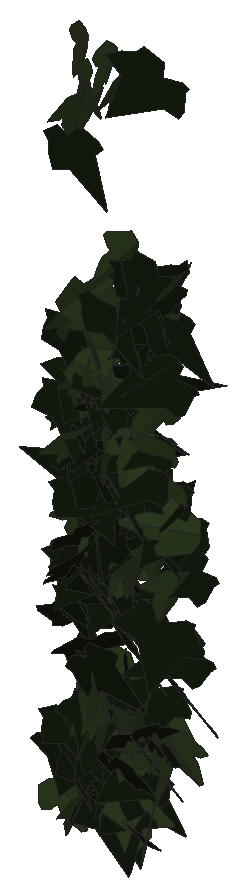
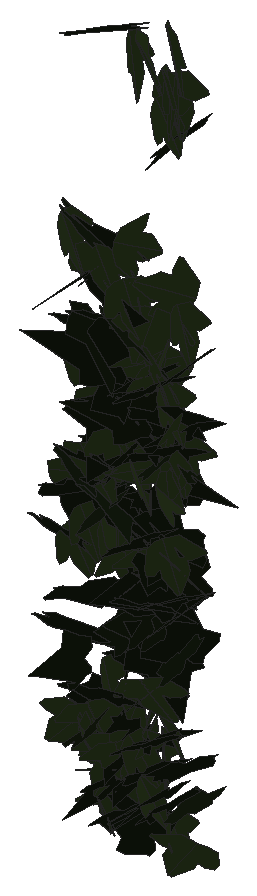
# SketchUp Ruby script. Lengths in inches.
U = 1.inch
M = Sketchup.active_model
def pt(a) = Geom::Point3d.new(a.map { |v| v * U })
def face(e, loops, mat)
  f = e.add_face(loops[0].map { |a| pt(a) })
  loops[1..].each { |l| e.add_face(l.map { |a| pt(a) }).erase! }
  f.material = f.back_material = mat if mat
  f
end
# faces: each face lists its corners as indices into pts; further lists are holes
def faces(e, pts, list, mat = nil) = list.each { |f| face(e, (f[0].is_a?(Array) ? f : [f]).map { |l| l.map { |i| pts[i] } }, mat) }
# xy, xz, yz: faces in a plane at the given z, y or x. An outline is a flat list of corners, or four numbers for a rectangle; further outlines are holes
def ring(l) = l.size == 4 ? [[l[0], l[1]], [l[2], l[1]], [l[2], l[3]], [l[0], l[3]]] : l.each_slice(2).to_a
def flat(e, list, mat, &to3) = list.each { |f| face(e, (f[0].is_a?(Array) ? f : [f]).map { |l| ring(l).map { |u, v| to3.(u, v) } }, mat) }
def xy(e, z, list, mat = nil) = flat(e, list, mat) { |x, y| [x, y, z] }
def xz(e, y, list, mat = nil) = flat(e, list, mat) { |x, z| [x, y, z] }
def yz(e, x, list, mat = nil) = flat(e, list, mat) { |y, z| [x, y, z] }
def lines(e, pts, list) = list.each { |a, b| e.add_line(pt(pts[a]), pt(pts[b])) }
# prism: a flat outline (further loops are holes) pulled along v
def prism(e, loops, v, mat = nil)
  f = face(e, loops, mat); d = Geom::Vector3d.new(v.map { |x| x * U })
  f.pushpull(f.normal.samedirection?(d) ? d.length : -d.length)
end
def box(e, o, s, mat = nil) = prism(e, [[o, [o[0] + s[0], o[1], o[2]], [o[0] + s[0], o[1] + s[1], o[2]], [o[0], o[1] + s[1], o[2]]]], [0, 0, s[2]], mat)
def at(x, y, z, deg = 0) = Geom::Transformation.translation(pt([x, y, z])) * Geom::Transformation.rotation(ORIGIN, Z_AXIS, deg.degrees)
def axes(o, x, y, z) = Geom::Transformation.new([*x, 0, *y, 0, *z, 0, *pt(o).to_a, 1])
def part(name) = M.definitions.add(name)
# library, detail: a bought-in or finely detailed component or shape, given as its bounding box
def library(name, o, s) = part(name).tap { |d| box(d.entities, o, s) }
def detail(e, o, s) = box(e.add_group.entities, o, s)
def put(e, d, t, mat = nil) = e.add_instance(d, t).tap { |i| i.material = mat if mat }
def group(e, t, mat = nil) = e.add_group.tap { |g| g.transformation = t; g.material = mat if mat }.entities
root = M.entities
M.materials.add("1026 AP 7946 SUNNY SIDE UP").color = [254, 231, 186]
M.materials.add("efeu1").color = [18, 25, 13]
M.materials.add("efeu2").color = [43, 57, 29]
c1 = part("ivyleaf_9")
p = [[1.54,2.16,1.25],[1.36,2.04,1.19],[-0.21,0.99,0.68],[-0.71,1.11,0.82],[-0.85,0.86,0.67],[-0.8,0.17,0.21],
  [-0.9,-0.01,0.1],[-0.67,-0.16,-0.02],[-0.08,-0.08,-0.05],[-0.03,-0.6,-0.4],[0.65,-0.88,-0.66],[0.83,-0.6,-0.49],
  [1.29,-0.42,-0.43],[1.8125,-0.07,-0.26],[1.21,0.44,0.15]]
faces(c1.entities,p,[[0,1,2,3,4,5,6,7,8,9,10,11,12,13,14]],"efeu1")
c2 = part("ivyleaf_10")
p = [[0,0.5,-0.03],[-0.0625,2.02,-0.43],[-0.19,2.01,-0.46],[-0.54,1.05,-0.29],[-0.52,0.625,-0.18],[-0.83,0.76,-0.28],
  [-1.16,0.64,-0.33],[-1.15,0.33,-0.24],[-0.77,-0.39,0.02],[-0.3,-0.51,0.16],[0.04,-0.48,0.23],[-0.02,2.01,-0.4375],
  [-0.06,2.01,-0.43],[0.04,-0.49,0.23],[0.67,-0.49,0.14],[1.38,0.36,-0.2],[1.375,0.51,-0.24],[0.81,0.65,-0.19],
  [0.62,0.59,-0.15],[0.6,1.09,-0.28],[0.5,1.23,-0.31]]
faces(c2.entities,p,[[0,1,2,3,4,5,6,7,8,9,10],[11,12,0,13,14,15,16,17,18,19,20]],"efeu2")
put(root,c1,axes([118.58,212.68,268.59],[-0.10148,-0.2145,0.16727],[0.05063,-0.17313,-0.22179],[0.42114,-0.03087,0.06697]),"1026 AP 7946 SUNNY SIDE UP")
put(root,c2,axes([118.54,212.65,268.07],[0.32447,0.10776,0.11567],[0.15112,0.05714,-0.23942],[-0.19158,0.22757,0.00705]),"1026 AP 7946 SUNNY SIDE UP")
put(root,c2,axes([118.68,212.77,274.12],[-0.06073,0.27731,-0.0585],[0.00468,-0.0585,-0.28874],[-0.44557,-0.03841,0.00494]),"1026 AP 7946 SUNNY SIDE UP")
put(root,c1,axes([118.59,212.76,274.85],[0.03448,-0.29512,0.03283],[-0.01092,-0.03414,-0.30491],[0.46691,0.021,-0.00956]),"1026 AP 7946 SUNNY SIDE UP")
put(root,c2,axes([118.8,212.83,272.25],[-0.18056,-0.25267,0.05829],[0.00801,-0.06563,-0.2845],[0.40755,-0.11065,0.03141]),"1026 AP 7946 SUNNY SIDE UP")
put(root,c2,axes([118.81,212.51,275.38],[-0.01092,-0.29639,-0.03515],[-0.00326,0.03249,-0.30522],[0.46882,-0.00667,-0.00294]),"1026 AP 7946 SUNNY SIDE UP")
put(root,c1,axes([118.55,212.8125,270.79],[0.18485,-0.24588,0.0457],[0.01515,-0.04607,-0.2808],[0.39297,0.11743,-0.01067]),"1026 AP 7946 SUNNY SIDE UP")
put(root,c1,axes([118.61,212.83,271.41],[0.05177,-0.27805,0.00823],[0.0003,-0.00961,-0.2885],[0.43746,0.03291,-0.00078]),"1026 AP 7946 SUNNY SIDE UP")
put(root,c2,axes([118.83,212.76,274.35],[0.00803,-0.29251,0.01042],[-0.01331,-0.01192,-0.30133],[0.46013,0.00476,-0.0089]),"1026 AP 7946 SUNNY SIDE UP")
put(root,c2,axes([118.9,212.65,278.67],[-0.31786,0.21972,0.09851],[-0.14415,0.04293,-0.30501],[-0.34729,-0.21892,0.03644]),"1026 AP 7946 SUNNY SIDE UP")
put(root,c1,axes([118.69,212.68,273.9],[-0.09442,-0.28697,-0.00864],[0.02044,0.00418,-0.30176],[0.45089,-0.06028,0.01187]),"1026 AP 7946 SUNNY SIDE UP")
put(root,c1,axes([118.91,212.89,274.19],[-0.3765,-0.16155,0.02026],[-0.00418,-0.03272,-0.29659],[0.25605,-0.23809,0.02495]),"1026 AP 7946 SUNNY SIDE UP")
put(root,c1,axes([118.6875,212.63,269.2],[0.01907,-0.25324,-0.11669],[0.04147,0.11249,-0.25882],[0.43332,0.00038,0.0299]),"1026 AP 7946 SUNNY SIDE UP")
put(root,c2,axes([118.9,212.44,273.5],[-0.12951,-0.28312,-0.0189],[0.01697,0.01429,-0.3036],[0.44563,-0.08283,0.00607]),"1026 AP 7946 SUNNY SIDE UP")
put(root,c2,axes([118.91,212.66,278.73],[0.19427,-0.27639,-0.07992],[-0.02868,0.07502,-0.31114],[0.44982,0.12415,0.01468]),"1026 AP 7946 SUNNY SIDE UP")
put(root,c2,axes([118.9,212.77,278.38],[0.00487,-0.30093,0.07367],[0.02675,-0.07295,-0.31003],[0.48625,0.00703,0.01632]),"1026 AP 7946 SUNNY SIDE UP")
put(root,c2,axes([118.91,212.58,279.31],[0.25386,-0.26163,-0.09519],[-0.02226,0.0973,-0.31379],[0.43496,0.15768,0.0395]),"1026 AP 7946 SUNNY SIDE UP")
put(root,c1,axes([118.9,212.77,271.46],[-0.25139,-0.19979,0.10642],[-0.01696,-0.1211,-0.25639],[0.35407,-0.14765,0.06328]),"1026 AP 7946 SUNNY SIDE UP")
put(root,c1,axes([118.85,212.57,270.75],[0.36294,0.1012,0.16315],[-0.24909,-0.02853,0.2574],[0.1576,-0.27814,0.0311]),"1026 AP 7946 SUNNY SIDE UP")
put(root,c2,axes([118.95,212.43,278.55],[-0.04065,-0.30751,-0.04097],[0.01889,0.03713,-0.31756],[0.48684,-0.02712,0.0089]),"1026 AP 7946 SUNNY SIDE UP")
put(root,c1,axes([119.32,212.4,273.06],[-0.2342,-0.03979,-0.26199],[-0.37431,-0.08981,0.15772],[-0.15306,0.2805,0.01517]),"1026 AP 7946 SUNNY SIDE UP")
put(root,c2,axes([118.89,212.77,273.02],[0.11866,-0.1923,0.20503],[0.10479,-0.18876,-0.21385],[0.42362,0.10055,-0.00453]),"1026 AP 7946 SUNNY SIDE UP")
put(root,c2,axes([118.98,212.4375,268.15],[0.03323,-0.2702,0.01416],[0.00097,-0.01527,-0.2793],[0.42554,0.02114,-0.00047]),"1026 AP 7946 SUNNY SIDE UP")
put(root,c1,axes([118.99,212.83,273.55],[-0.26978,-0.23022,0.03448],[-0.00865,-0.03917,-0.29538],[0.366,-0.17062,0.01843]),"1026 AP 7946 SUNNY SIDE UP")
put(root,c1,axes([118.84,212.17,271.6],[0.19476,0.04727,0.25703],[0.24352,0.20557,-0.11826],[-0.3159,0.18761,0.0673]),"1026 AP 7946 SUNNY SIDE UP")
put(root,c1,axes([118.87,212.7,268.61],[0.02193,-0.27626,-0.0293],[-0.01072,0.02655,-0.28476],[0.43632,0.01454,-0.00552]),"1026 AP 7946 SUNNY SIDE UP")
put(root,c1,axes([118.85,212.42,277.9375],[0.13716,-0.27594,-0.10569],[-0.04552,0.0968,-0.29757],[0.45981,0.0919,0.00207]),"1026 AP 7946 SUNNY SIDE UP")
put(root,c1,axes([119.17,212.46,270.58],[0.06548,0.26201,-0.10257],[-0.03676,-0.09857,-0.27379],[-0.44004,0.04722,0.00761]),"1026 AP 7946 SUNNY SIDE UP")
put(root,c1,axes([119.01,212.26,273.3],[-0.19086,0.27196,-0.01341],[0.00514,0.01739,0.30674],[0.42821,0.12101,-0.00966]),"1026 AP 7946 SUNNY SIDE UP")
put(root,c1,axes([119.04,212.26,272.2],[0.18811,0.23917,0.09452],[0.07675,0.0766,-0.2749],[-0.39464,0.1289,-0.00841]),"1026 AP 7946 SUNNY SIDE UP")
put(root,c2,axes([118.99,212.32,275.57],[-0.03665,-0.15773,0.27901],[0.03852,0.27073,0.16564],[-0.49253,0.03291,-0.00781]),"1026 AP 7946 SUNNY SIDE UP")
put(root,c1,axes([119.17,212.65,271.99],[-0.1635,0.17125,-0.20163],[0.12844,-0.17971,-0.20672],[-0.38944,-0.13116,0.01647]),"1026 AP 7946 SUNNY SIDE UP")
put(root,c1,axes([119.28,212.65,272.125],[-0.41933,0.08612,-0.02938],[0.02968,-0.03548,-0.28749],[-0.13977,-0.2659,0.0271]),"1026 AP 7946 SUNNY SIDE UP")
put(root,c2,axes([119.05,212.68,273.6],[0.42207,-0.09618,-0.00233],[-0.01596,-0.02327,-0.29272],[0.15041,0.26742,-0.02452]),"1026 AP 7946 SUNNY SIDE UP")
put(root,c2,axes([119.125,212.8125,270.22],[0.36804,0.09952,-0.10881],[-0.14682,-0.05156,-0.26212],[-0.17553,0.2518,-0.0089]),"1026 AP 7946 SUNNY SIDE UP")
put(root,c2,axes([119.12,212.81,268.79],[0.02146,-0.25286,0.07339],[0.00072,-0.07275,-0.26128],[0.41369,0.01324,-0.00335]),"1026 AP 7946 SUNNY SIDE UP")
put(root,c1,axes([118.92,212.7,268.75],[0.18081,-0.19196,-0.17184],[-0.04871,0.16996,-0.22397],[0.39576,0.10862,0.05094]),"1026 AP 7946 SUNNY SIDE UP")
put(root,c1,axes([119.13,212.82,269.02],[-0.19573,-0.20834,0.09507],[-0.06147,-0.08544,-0.25033],[0.35375,-0.13012,0.0091]),"1026 AP 7946 SUNNY SIDE UP")
put(root,c1,axes([118.97,212.89,270.26],[0.03992,-0.26487,0.05518],[-0.00324,-0.0555,-0.27434],[0.42538,0.02443,-0.00727]),"1026 AP 7946 SUNNY SIDE UP")
put(root,c1,axes([118.87,212.83,271.2],[0.24445,-0.2175,0.07178],[0.04949,-0.06458,-0.27554],[0.35629,0.1582,-0.01097]),"1026 AP 7946 SUNNY SIDE UP")
put(root,c2,axes([119.16,212.41,269.27],[0.10542,-0.24459,-0.1297],[-0.00143,0.12797,-0.25874],[0.43156,0.06017,0.03083]),"1026 AP 7946 SUNNY SIDE UP")
put(root,c1,axes([118.93,212.6875,273.5],[0.26532,-0.2202,-0.0903],[-0.04809,0.08493,-0.28402],[0.36882,0.16948,0.02792]),"1026 AP 7946 SUNNY SIDE UP")
put(root,c2,axes([119.27,212.66,274.74],[0.20544,-0.20687,-0.15928],[-0.15272,0.11978,-0.25086],[0.3751,0.16207,-0.0149]),"1026 AP 7946 SUNNY SIDE UP")
put(root,c2,axes([119.09,212.54,274.94],[-0.21051,0.25398,-0.05746],[0.03298,-0.05361,-0.29601],[-0.40804,-0.13536,0.00572]),"1026 AP 7946 SUNNY SIDE UP")
put(root,c2,axes([119.23,212.39,269.61],[0.25938,-0.20632,-0.07883],[-0.09868,0.04603,-0.27112],[0.33098,0.17541,-0.01905]),"1026 AP 7946 SUNNY SIDE UP")
put(root,c1,axes([119.13,212.65,269.4],[-0.16533,-0.24244,0.04077],[-0.00673,-0.04272,-0.27216],[0.38655,-0.10444,0.0127]),"1026 AP 7946 SUNNY SIDE UP")
put(root,c1,axes([119.18,212.85,271.35],[-0.33244,-0.1684,-0.06579],[0.12306,0.00121,-0.27428],[0.25447,-0.22058,0.04668]),"1026 AP 7946 SUNNY SIDE UP")
put(root,c1,axes([119.09,212.91,269.47],[-0.10931,-0.25655,0.01204],[0.04968,-0.02205,-0.2714],[0.40086,-0.06722,0.03692]),"1026 AP 7946 SUNNY SIDE UP")
put(root,c1,axes([119.14,212.8125,274.4],[-0.15244,-0.27137,0.05732],[0.00506,-0.06167,-0.29625],[0.43604,-0.09416,0.02347]),"1026 AP 7946 SUNNY SIDE UP")
put(root,c2,axes([119.18,212.66,275.29],[-0.3818,-0.16452,-0.06141],[0.12487,-0.01448,-0.29679],[0.24463,-0.24938,0.05565]),"1026 AP 7946 SUNNY SIDE UP")
put(root,c2,axes([119.1875,212.6,274.59],[0.06134,0.27653,-0.08104],[-0.05979,-0.07531,-0.28689],[-0.44879,0.04783,0.02714]),"1026 AP 7946 SUNNY SIDE UP")
put(root,c2,axes([118.94,212.64,273.3],[-0.13355,-0.07805,-0.27428],[0.39461,0.09604,-0.11111],[0.18444,-0.26199,0.0391]),"1026 AP 7946 SUNNY SIDE UP")
put(root,c2,axes([119.21,212.76,279.11],[0.27061,-0.25999,0.04793],[0.02709,-0.04613,-0.32128],[0.41484,0.17261,-0.01028]),"1026 AP 7946 SUNNY SIDE UP")
put(root,c2,axes([119.3,212.8,269.32],[-0.05993,-0.25485,0.08837],[-0.02874,-0.08545,-0.26591],[0.42257,-0.04196,-0.00555]),"1026 AP 7946 SUNNY SIDE UP")
put(root,c2,axes([119.26,212.51,274.42],[0.33919,-0.18615,-0.03514],[-0.0489,0.01453,-0.2933],[0.29324,0.21775,-0.00826]),"1026 AP 7946 SUNNY SIDE UP")
put(root,c2,axes([119.1875,212.68,272.01],[0.20738,0.2401,-0.04856],[-0.01317,-0.05063,-0.28198],[-0.38493,0.13109,-0.01651]),"1026 AP 7946 SUNNY SIDE UP")
put(root,c1,axes([118.96,212.65,271.63],[0.4236,-0.02141,0.0859],[0.12889,-0.02116,-0.27816],[0.04195,0.28124,-0.01272]),"1026 AP 7946 SUNNY SIDE UP")
put(root,c1,axes([119.06,212.46,272.82],[-0.0129,-0.23668,-0.17327],[0.10554,0.16081,-0.23747],[0.44292,-0.04521,0.05154]),"1026 AP 7946 SUNNY SIDE UP")
put(root,c2,axes([119.33,212.4,269.41],[0.07074,-0.07671,-0.27977],[0.02194,0.27483,-0.07611],[0.44252,-0.00136,0.04849]),"1026 AP 7946 SUNNY SIDE UP")
put(root,c2,axes([119.33,212.76,273.21],[0.14434,-0.2762,0.01395],[0.00846,-0.01413,-0.29992],[0.43487,0.09195,0.0012]),"1026 AP 7946 SUNNY SIDE UP")
put(root,c1,axes([119.59,212.28,272.02],[-0.04798,0.10117,0.30367],[-0.20254,0.26497,-0.10608],[-0.44528,-0.13142,0.01553]),"1026 AP 7946 SUNNY SIDE UP")
put(root,c2,axes([119.51,212.39,273.15],[-0.24806,0.15581,0.2064],[-0.2529,0.11977,-0.22673],[-0.30731,-0.22434,0.01998]),"1026 AP 7946 SUNNY SIDE UP")
put(root,c2,axes([119.3,212.34,269.9375],[0.11206,-0.21982,-0.16627],[0.08462,0.17368,-0.2199],[0.41919,0.0237,0.08884]),"1026 AP 7946 SUNNY SIDE UP")
put(root,c1,axes([119.48,212.57,274.16],[0.13879,0.25151,-0.1236],[-0.1024,-0.10528,-0.27408],[-0.42704,0.10699,0.02555]),"1026 AP 7946 SUNNY SIDE UP")
put(root,c1,axes([119.26,212.67,274.46],[-0.03376,-0.29447,-0.02081],[0.01633,0.01781,-0.30392],[0.46366,-0.02207,0.00919]),"1026 AP 7946 SUNNY SIDE UP")
put(root,c2,axes([119.13,212.42,274.64],[-0.14289,-0.11409,-0.26965],[0.39928,0.09191,-0.13188],[0.20326,-0.26074,0.06949]),"1026 AP 7946 SUNNY SIDE UP")
put(root,c1,axes([119.15,212.75,271.13],[0.26787,-0.2088,0.06411],[0.03774,-0.06203,-0.27721],[0.34105,0.17087,-0.01968]),"1026 AP 7946 SUNNY SIDE UP")
put(root,c2,axes([119.47,212.76,275.63],[-0.20217,-0.26545,0.06075],[0.0069,-0.0689,-0.30232],[0.42803,-0.12427,0.03357]),"1026 AP 7946 SUNNY SIDE UP")
put(root,c1,axes([119.375,212.83,272.15],[-0.17087,-0.24373,0.09093],[-0.02084,-0.09185,-0.27434],[0.40781,-0.10682,0.02408]),"1026 AP 7946 SUNNY SIDE UP")
put(root,c2,axes([119.45,212.82,276.32],[-0.00921,-0.12799,0.29569],[0.05921,-0.28602,-0.13195],[0.49165,0.03205,0.02143]),"1026 AP 7946 SUNNY SIDE UP")
put(root,c1,axes([119.32,212.74,273.52],[0.13451,-0.24198,-0.13025],[-0.08259,0.11397,-0.26352],[0.42026,0.09984,-0.0101]),"1026 AP 7946 SUNNY SIDE UP")
put(root,c1,axes([119.3,212.75,271.62],[0.06004,-0.27427,0.04607],[0.0032,-0.04643,-0.28552],[0.43735,0.038,-0.00423]),"1026 AP 7946 SUNNY SIDE UP")
put(root,c1,axes([119.72,212.73,275.18],[-0.34567,0.19063,-0.03887],[0.01916,-0.04497,-0.29885],[-0.3053,-0.21866,0.02526]),"1026 AP 7946 SUNNY SIDE UP")
put(root,c2,axes([119.53,212.57,278.99],[0.07579,-0.30265,-0.08662],[0.01276,0.08451,-0.31451],[0.49303,0.04434,0.02145]),"1026 AP 7946 SUNNY SIDE UP")
put(root,c1,axes([119.16,212.42,270.3],[0.0599,-0.06791,-0.27882],[0.41852,0.08966,0.01597],[0.12978,-0.25779,0.07721]),"1026 AP 7946 SUNNY SIDE UP")
put(root,c1,axes([119.33,212.5,275.6],[0.14335,-0.27834,-0.06651],[0.00259,0.06663,-0.3005],[0.44872,0.08854,0.02298]),"1026 AP 7946 SUNNY SIDE UP")
put(root,c2,axes([119.47,212.74,273.46],[0.44706,-0.02368,0.01942],[0.02554,-0.03237,-0.29238],[0.04031,0.2831,-0.03012]),"1026 AP 7946 SUNNY SIDE UP")
put(root,c2,axes([119.625,212.44,275.45],[0.19034,-0.26275,-0.10795],[-0.0171,0.10796,-0.29543],[0.4436,0.1169,0.03493]),"1026 AP 7946 SUNNY SIDE UP")
put(root,c2,axes([119.6,212.21,273.64],[0.09441,-0.15575,-0.24558],[0.03101,0.24444,-0.15858],[0.4455,0.01599,0.06308]),"1026 AP 7946 SUNNY SIDE UP")
put(root,c1,axes([119.25,212.58,268],[0.15529,-0.14983,0.23424],[0.26526,-0.15733,-0.18253],[0.33753,0.19258,0.03568]),"1026 AP 7946 SUNNY SIDE UP")
put(root,c2,axes([119.625,212.74,273.49],[-0.35192,-0.18721,0.02357],[0.06013,-0.08135,-0.28751],[0.29061,-0.20987,0.08803]),"1026 AP 7946 SUNNY SIDE UP")
put(root,c2,axes([119.64,212.63,271.85],[0.14403,0.23689,-0.13203],[-0.12223,-0.10783,-0.26046],[-0.40654,0.11635,0.03153]),"1026 AP 7946 SUNNY SIDE UP")
put(root,c2,axes([119.62,212.5,269.59],[-0.34487,0.14505,-0.02712],[0.01592,-0.03372,-0.2701],[-0.23148,-0.21841,0.02183]),"1026 AP 7946 SUNNY SIDE UP")
put(root,c1,axes([119.59,212.64,268.21],[-0.14865,-0.16689,0.18263],[-0.03199,-0.18507,-0.19074],[0.38259,-0.08032,0.05501]),"1026 AP 7946 SUNNY SIDE UP")
put(root,c1,axes([119.26,212.78,273.97],[0.32138,-0.14486,0.15688],[0.2276,-0.05857,-0.25649],[0.24092,0.24857,0.03303]),"1026 AP 7946 SUNNY SIDE UP")
put(root,c1,axes([119.42,212.42,273.15],[0.26462,-0.22616,-0.04853],[-0.03195,0.04197,-0.29004],[0.36144,0.16929,0.00989]),"1026 AP 7946 SUNNY SIDE UP")
put(root,c1,axes([119.45,212.85,270.1],[0.03838,-0.06702,-0.26775],[0.34973,-0.14036,0.05807],[-0.2352,-0.21965,0.04266]),"1026 AP 7946 SUNNY SIDE UP")
put(root,c2,axes([119.625,212.79,269.17],[0.24193,0.20676,-0.04875],[-0.03868,-0.04213,-0.2657],[-0.33169,0.15572,-0.00458]),"1026 AP 7946 SUNNY SIDE UP")
put(root,c1,axes([119.54,212.47,268.25],[-0.24382,-0.16713,-0.17717],[0.23238,0.09328,-0.23138],[0.2956,-0.21118,0.03577]),"1026 AP 7946 SUNNY SIDE UP")
put(root,c1,axes([119.625,212.36,268.98],[0.38435,0.00528,-0.12955],[-0.19726,-0.01265,-0.25178],[-0.01647,0.27461,-0.0075]),"1026 AP 7946 SUNNY SIDE UP")
put(root,c1,axes([119.65,212.58,269.44],[0.38059,0.00846,-0.14363],[-0.21767,-0.02334,-0.2491],[-0.02982,0.27837,-0.01488]),"1026 AP 7946 SUNNY SIDE UP")
put(root,c1,axes([120,212.55,275.2],[-0.03232,0.06974,0.31721],[-0.2284,0.27144,-0.07182],[-0.44008,-0.14599,0.01398]),"1026 AP 7946 SUNNY SIDE UP")
put(root,c1,axes([119.95,212.57,272.53],[0.01252,0.23703,0.16214],[-0.16358,0.14767,-0.22476],[-0.41516,-0.05104,0.09345]),"1026 AP 7946 SUNNY SIDE UP")
put(root,c1,axes([119.58,212.69,273.14],[0.0359,-0.28333,0.02515],[-0.00266,-0.02624,-0.29295],[0.44737,0.02258,-0.00376]),"1026 AP 7946 SUNNY SIDE UP")
put(root,c1,axes([119.625,212.65,268.22],[-0.04354,-0.25766,-0.04082],[0.0233,0.03675,-0.26653],[0.4089,-0.02953,0.01084]),"1026 AP 7946 SUNNY SIDE UP")
put(root,c1,axes([119.71,212.48,273.65],[0.37289,0.20312,-0.01283],[0.0074,-0.02636,-0.32095],[-0.32001,0.23607,-0.02238]),"1026 AP 7946 SUNNY SIDE UP")
put(root,c2,axes([119.75,212.77,269.24],[0.2415,0.21018,-0.03476],[-0.02735,-0.03055,-0.26832],[-0.33391,0.15451,-0.00316]),"1026 AP 7946 SUNNY SIDE UP")
put(root,c2,axes([119.98,212.74,275.95],[-0.42218,0.04392,0.1091],[-0.17847,-0.06824,-0.26833],[-0.02271,-0.28035,0.08063]),"1026 AP 7946 SUNNY SIDE UP")
put(root,c1,axes([119.57,212.56,270.81],[0.29522,-0.19475,0.03536],[0.01738,-0.03843,-0.27825],[0.31076,0.18716,-0.01802]),"1026 AP 7946 SUNNY SIDE UP")
put(root,c2,axes([119.85,212.43,275.91],[0.18727,-0.27706,-0.03188],[-0.02772,0.02439,-0.31046],[0.43721,0.12022,-0.00603]),"1026 AP 7946 SUNNY SIDE UP")
put(root,c1,axes([119.93,212.58,273.32],[-0.38401,-0.14584,0.0359],[-0.02847,-0.03902,-0.29222],[0.23435,-0.24371,0.02333]),"1026 AP 7946 SUNNY SIDE UP")
put(root,c1,axes([119.91,212.72,268.74],[-0.34179,-0.12394,0.10679],[-0.03736,-0.14836,-0.23336],[0.25203,-0.19009,0.11023]),"1026 AP 7946 SUNNY SIDE UP")
put(root,c1,axes([119.63,212.79,276.06],[0.13496,-0.28405,-0.0577],[-0.00965,0.05494,-0.3052],[0.45465,0.08548,0.01065]),"1026 AP 7946 SUNNY SIDE UP")
put(root,c1,axes([119.99,212.64,273.83],[-0.39695,-0.12739,0.0551],[-0.05233,-0.05358,-0.28972],[0.2113,-0.25258,0.03175]),"1026 AP 7946 SUNNY SIDE UP")
put(root,c2,axes([119.79,212.59,268.9],[0.16903,0.19835,0.1413],[-0.00606,0.1504,-0.22191],[-0.37814,0.08626,0.06672]),"1026 AP 7946 SUNNY SIDE UP")
put(root,c2,axes([119.93,212.52,272.01],[-0.01413,-0.29293,0.03143],[0.00013,-0.03219,-0.3021],[0.46337,-0.00892,0.00104]),"1026 AP 7946 SUNNY SIDE UP")
put(root,c2,axes([120.06,212.5,273.8],[-0.41041,-0.07323,0.09961],[-0.13802,-0.0457,-0.27885],[0.13236,-0.27471,0.01807]),"1026 AP 7946 SUNNY SIDE UP")
put(root,c1,axes([120.15,212.65,272.58],[0.09409,0.03219,-0.30355],[-0.30347,-0.22417,-0.06688],[-0.35412,0.20065,-0.02335]),"1026 AP 7946 SUNNY SIDE UP")
put(root,c2,axes([119.84,212.46,268.31],[0.3178,0.21164,-0.02486],[-0.00977,-0.02904,-0.30122],[-0.33501,0.20161,-0.0148]),"1026 AP 7946 SUNNY SIDE UP")
put(root,c2,axes([119.91,212.47,273.78],[0.25532,0.22042,-0.10829],[-0.07858,-0.0951,-0.28217],[-0.37673,0.16922,-0.01454]),"1026 AP 7946 SUNNY SIDE UP")
put(root,c2,axes([119.84,212.58,271.87],[0.03323,-0.1723,-0.23499],[0.04254,-0.22551,0.17752],[-0.44624,-0.03433,-0.00058]),"1026 AP 7946 SUNNY SIDE UP")
put(root,c1,axes([119.79,212.64,268.5625],[0.11357,-0.17004,-0.19405],[-0.02731,0.19109,-0.18441],[0.39695,0.0618,0.04283]),"1026 AP 7946 SUNNY SIDE UP")
put(root,c1,axes([119.93,212.88,269.92],[-0.31931,-0.1625,-0.07669],[0.15097,-0.00571,-0.26025],[0.23635,-0.2159,0.06263]),"1026 AP 7946 SUNNY SIDE UP")
put(root,c1,axes([119.77,212.83,272.49],[0.17049,-0.26104,0.01466],[0.02567,-0.01022,-0.29103],[0.41039,0.10908,0.01211]),"1026 AP 7946 SUNNY SIDE UP")
put(root,c1,axes([119.98,212.31,269.52],[0.21482,0.23922,0.02031],[0.03361,0.0089,-0.28337],[-0.37575,0.13756,-0.01374]),"1026 AP 7946 SUNNY SIDE UP")
put(root,c1,axes([120.08,212.75,279.11],[-0.34778,-0.17877,0.13288],[-0.0504,-0.15602,-0.27813],[0.34389,-0.20366,0.09362]),"1026 AP 7946 SUNNY SIDE UP")
put(root,c2,axes([120.01,212.61,269.43],[-0.12225,-0.24899,-0.08702],[0.08634,0.06928,-0.2665],[0.40359,-0.09024,0.03066]),"1026 AP 7946 SUNNY SIDE UP")
put(root,c2,axes([120.04,212.78,269.57],[0.29199,0.17355,-0.09259],[-0.10355,-0.0626,-0.26221],[-0.2901,0.19703,0.00041]),"1026 AP 7946 SUNNY SIDE UP")
put(root,c1,axes([120.17,212.47,274.84],[-0.01997,0.29535,0.01209],[0.00793,0.01028,-0.30444],[-0.46462,-0.01252,-0.00572]),"1026 AP 7946 SUNNY SIDE UP")
put(root,c2,axes([120.125,212.72,273.1],[0.40682,-0.01171,-0.12112],[-0.17535,0.0688,-0.25963],[0.06104,0.2757,0.06136]),"1026 AP 7946 SUNNY SIDE UP")
put(root,c1,axes([120.12,212.59,276.22],[-0.44659,-0.04931,-0.09741],[0.15334,-0.01322,-0.29562],[0.06688,-0.29896,0.02734]),"1026 AP 7946 SUNNY SIDE UP")
put(root,c2,axes([120.08,212.39,269.93],[0.05648,-0.26704,-0.02823],[0.0106,0.02701,-0.27722],[0.42173,0.03508,0.01075]),"1026 AP 7946 SUNNY SIDE UP")
put(root,c1,axes([120.1875,212.79,273.08],[-0.43845,-0.05086,-0.03933],[0.06549,-0.01799,-0.29097],[0.07522,-0.28083,0.02406]),"1026 AP 7946 SUNNY SIDE UP")
put(root,c1,axes([120.13,212.92,269.2],[0.10636,-0.25662,-0.01311],[0.01025,-0.00994,0.27332],[-0.40377,-0.06785,0.00349]),"1026 AP 7946 SUNNY SIDE UP")
put(root,c2,axes([120.12,212.77,272.24],[-0.09291,-0.27349,0.04442],[0.01171,-0.04723,-0.28799],[0.43558,-0.05706,0.01722]),"1026 AP 7946 SUNNY SIDE UP")
put(root,c1,axes([119.82,212.48,269.33],[0.33601,-0.16773,0.04211],[0.02987,-0.04333,-0.27919],[0.27018,0.21339,-0.02151]),"1026 AP 7946 SUNNY SIDE UP")
put(root,c2,axes([120.01,212.59,268.17],[0.22204,-0.20056,0.1214],[0.11904,-0.09213,-0.2531],[0.34682,0.16003,0.00915]),"1026 AP 7946 SUNNY SIDE UP")
put(root,c1,axes([119.75,212.67,274.52],[0.18174,-0.01555,0.27862],[0.42571,0.01927,-0.1179],[-0.01832,0.29357,0.02423]),"1026 AP 7946 SUNNY SIDE UP")
put(root,c2,axes([120.27,212.58,274.4],[-0.16736,-0.22663,0.15989],[-0.06776,-0.152,-0.25786],[0.42772,-0.11276,0.02171]),"1026 AP 7946 SUNNY SIDE UP")
put(root,c2,axes([120.1,212.8,269.36],[0.0991,-0.17466,0.19637],[0.1171,-0.17668,-0.19219],[0.3905,0.09731,0.0078]),"1026 AP 7946 SUNNY SIDE UP")
put(root,c1,axes([120.43,212.7,272.94],[-0.29714,0.21144,-0.02341],[0.00411,-0.02969,-0.29174],[-0.33457,-0.18816,0.01721]),"1026 AP 7946 SUNNY SIDE UP")
put(root,c1,axes([120.45,212.55,274.85],[-0.42279,-0.07493,0.1051],[-0.12727,-0.08362,-0.28236],[0.15373,-0.27532,0.05528]),"1026 AP 7946 SUNNY SIDE UP")
put(root,c1,axes([120.5,212.55,276.26],[-0.37416,0.17277,-0.05315],[0.03495,-0.05829,-0.3013],[-0.28181,-0.23662,0.0332]),"1026 AP 7946 SUNNY SIDE UP")
put(root,c1,axes([120.36,212.85,272.64],[-0.32407,-0.18824,0.04711],[-0.03304,-0.04622,-0.2871],[0.3032,-0.20623,0.01908]),"1026 AP 7946 SUNNY SIDE UP")
put(root,c2,axes([120.58,212.58,272.62],[-0.04733,0.10728,0.28348],[-0.3065,-0.21428,0.06298],[0.3477,-0.17428,0.09411]),"1026 AP 7946 SUNNY SIDE UP")
put(root,c1,axes([120.5625,212.84,270.68],[-0.41172,-0.00747,0.07631],[-0.11278,-0.04778,-0.2663],[0.03159,-0.2679,0.04375]),"1026 AP 7946 SUNNY SIDE UP")
put(root,c1,axes([120.3,212.625,271.13],[-0.2359,-0.27236,0.01118],[0.01488,-0.01935,-0.31993],[0.42844,-0.14929,0.01727]),"1026 AP 7946 SUNNY SIDE UP")
put(root,c2,axes([120.4,212.77,276.25],[0.04562,-0.30164,0.0116],[0.00155,-0.01294,-0.31225],[0.47473,0.02903,-0.0001]),"1026 AP 7946 SUNNY SIDE UP")
put(root,c2,axes([120.42,212.63,271.83],[-0.12754,-0.26381,0.09144],[0.01323,-0.09627,-0.28266],[0.43822,-0.07387,0.03515]),"1026 AP 7946 SUNNY SIDE UP")
put(root,c1,axes([120.2,212.66,275.59],[0.19584,-0.24139,-0.13353],[-0.02261,0.13495,-0.27527],[0.4292,0.11725,0.04643]),"1026 AP 7946 SUNNY SIDE UP")
put(root,c2,axes([120.44,212.4,269.04],[0.18003,-0.25194,-0.04963],[-0.02387,0.04444,-0.28479],[0.40221,0.11541,0.00531]),"1026 AP 7946 SUNNY SIDE UP")
put(root,c2,axes([120.29,212.76,269.36],[-0.36239,0.06014,-0.13419],[0.18379,-0.06532,-0.24387],[-0.13166,-0.25672,0.02893]),"1026 AP 7946 SUNNY SIDE UP")
put(root,c1,axes([120.17,212.8,270.24],[0.33386,-0.15711,0.0315],[0.01913,-0.03629,-0.27139],[0.25122,0.21155,-0.0212]),"1026 AP 7946 SUNNY SIDE UP")
put(root,c1,axes([120.67,212.8,271.97],[-0.43319,0.03873,0.01541],[-0.03086,-0.03469,-0.28426],[-0.05739,-0.2737,0.03655]),"1026 AP 7946 SUNNY SIDE UP")
